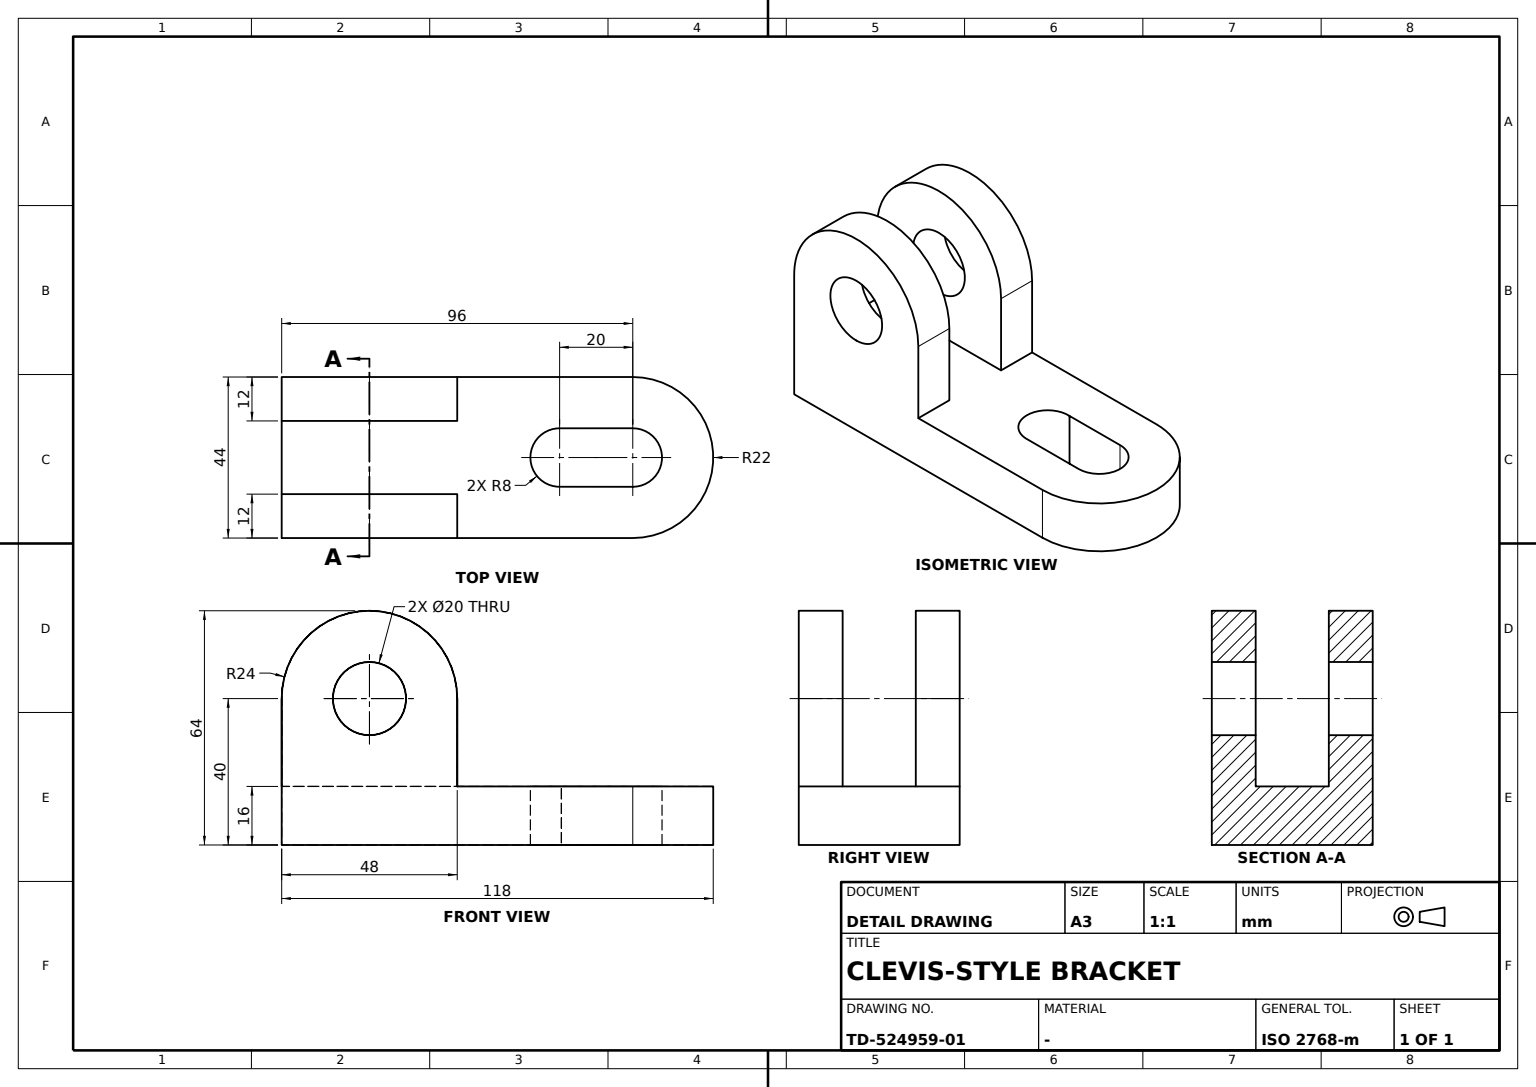
ISO-10303-21;
HEADER;
FILE_DESCRIPTION((''),'2;1');
FILE_NAME('','',(''),(''),'','','');
FILE_SCHEMA(('AUTOMOTIVE_DESIGN'));
ENDSEC;
DATA;
#1=APPLICATION_CONTEXT('');
#2=PRODUCT_CONTEXT('',#1,'mechanical');
#3=PRODUCT('','','',(#2));
#4=PRODUCT_DEFINITION_FORMATION('','',#3);
#5=PRODUCT_DEFINITION_CONTEXT('',#1,'design');
#6=PRODUCT_DEFINITION('','',#4,#5);
#7=PRODUCT_DEFINITION_SHAPE('','',#6);
#8=(LENGTH_UNIT()NAMED_UNIT(*)SI_UNIT(.MILLI.,.METRE.));
#9=(NAMED_UNIT(*)PLANE_ANGLE_UNIT()SI_UNIT($,.RADIAN.));
#10=(NAMED_UNIT(*)SI_UNIT($,.STERADIAN.)SOLID_ANGLE_UNIT());
#11=UNCERTAINTY_MEASURE_WITH_UNIT(LENGTH_MEASURE(0.005),#8,'distance_accuracy_value','');
#12=(GEOMETRIC_REPRESENTATION_CONTEXT(3)GLOBAL_UNCERTAINTY_ASSIGNED_CONTEXT((#11))GLOBAL_UNIT_ASSIGNED_CONTEXT((#8,#9,#10))REPRESENTATION_CONTEXT('',''));
#13=CARTESIAN_POINT('',(0.,-10.,40.));
#14=VERTEX_POINT('',#13);
#15=CARTESIAN_POINT('',(0.,-10.,16.));
#16=VERTEX_POINT('',#15);
#17=DIRECTION('',(0.,0.,-1.));
#18=VECTOR('',#17,1000.);
#19=LINE('',#13,#18);
#20=EDGE_CURVE('',#14,#16,#19,.T.);
#21=ORIENTED_EDGE('',*,*,#20,.F.);
#22=CARTESIAN_POINT('',(0.,-22.,40.));
#23=VERTEX_POINT('',#22);
#24=CARTESIAN_POINT('',(0.,16.,40.));
#25=DIRECTION('',(0.,1.,0.));
#26=VECTOR('',#25,1000.);
#27=LINE('',#24,#26);
#28=EDGE_CURVE('',#23,#14,#27,.T.);
#29=ORIENTED_EDGE('',*,*,#28,.F.);
#30=CARTESIAN_POINT('',(0.,-22.,16.));
#31=VERTEX_POINT('',#30);
#32=CARTESIAN_POINT('',(0.,-22.,0.));
#33=LINE('',#32,#18);
#34=EDGE_CURVE('',#23,#31,#33,.T.);
#35=ORIENTED_EDGE('',*,*,#34,.T.);
#36=CARTESIAN_POINT('',(0.,22.,16.));
#37=LINE('',#36,#26);
#38=EDGE_CURVE('',#31,#16,#37,.T.);
#39=ORIENTED_EDGE('',*,*,#38,.T.);
#40=EDGE_LOOP('',(#21,#29,#35,#39));
#41=FACE_BOUND('',#40,.T.);
#42=CARTESIAN_POINT('',(0.,22.,40.));
#43=DIRECTION('',(-1.,0.,0.));
#44=AXIS2_PLACEMENT_3D('',#42,#43,#17);
#45=PLANE('',#44);
#46=ADVANCED_FACE('',(#41),#45,.F.);
#47=CARTESIAN_POINT('',(-24.,10.,50.));
#48=VERTEX_POINT('',#47);
#49=CARTESIAN_POINT('',(-24.,10.,40.));
#50=DIRECTION('',(0.,0.,1.));
#51=AXIS2_PLACEMENT_3D('',#49,#25,#50);
#52=CIRCLE('',#51,10.);
#53=EDGE_CURVE('',#48,#48,#52,.T.);
#54=ORIENTED_EDGE('',*,*,#53,.T.);
#55=EDGE_LOOP('',(#54));
#56=FACE_BOUND('',#55,.T.);
#57=CARTESIAN_POINT('',(-48.,10.,16.));
#58=VERTEX_POINT('',#57);
#59=CARTESIAN_POINT('',(-48.,10.,40.));
#60=VERTEX_POINT('',#59);
#61=CARTESIAN_POINT('',(-48.,10.,0.));
#62=VECTOR('',#50,1000.);
#63=LINE('',#61,#62);
#64=EDGE_CURVE('',#58,#60,#63,.T.);
#65=ORIENTED_EDGE('',*,*,#64,.F.);
#66=CARTESIAN_POINT('',(0.,10.,16.));
#67=VERTEX_POINT('',#66);
#68=VECTOR('',#43,1000.);
#69=LINE('',#66,#68);
#70=EDGE_CURVE('',#67,#58,#69,.T.);
#71=ORIENTED_EDGE('',*,*,#70,.F.);
#72=CARTESIAN_POINT('',(0.,10.,40.));
#73=VERTEX_POINT('',#72);
#74=LINE('',#72,#18);
#75=EDGE_CURVE('',#73,#67,#74,.T.);
#76=ORIENTED_EDGE('',*,*,#75,.F.);
#77=CIRCLE('',#51,24.);
#78=EDGE_CURVE('',#60,#73,#77,.T.);
#79=ORIENTED_EDGE('',*,*,#78,.F.);
#80=EDGE_LOOP('',(#65,#71,#76,#79));
#81=FACE_BOUND('',#80,.T.);
#82=CARTESIAN_POINT('',(0.,10.,0.));
#83=AXIS2_PLACEMENT_3D('',#82,#25,#43);
#84=PLANE('',#83);
#85=ADVANCED_FACE('',(#56,#81),#84,.F.);
#86=CARTESIAN_POINT('',(48.,22.,0.));
#87=VERTEX_POINT('',#86);
#88=CARTESIAN_POINT('',(48.,22.,16.));
#89=VERTEX_POINT('',#88);
#90=CARTESIAN_POINT('',(48.,22.,8.));
#91=LINE('',#90,#62);
#92=EDGE_CURVE('',#87,#89,#91,.T.);
#93=ORIENTED_EDGE('',*,*,#92,.T.);
#94=CARTESIAN_POINT('',(48.,-22.,16.));
#95=VERTEX_POINT('',#94);
#96=CARTESIAN_POINT('',(48.,0.,16.));
#97=DIRECTION('',(1.,0.,0.));
#98=AXIS2_PLACEMENT_3D('',#96,#50,#97);
#99=CIRCLE('',#98,22.);
#100=EDGE_CURVE('',#95,#89,#99,.T.);
#101=ORIENTED_EDGE('',*,*,#100,.F.);
#102=CARTESIAN_POINT('',(48.,-22.,0.));
#103=VERTEX_POINT('',#102);
#104=CARTESIAN_POINT('',(48.,-22.,8.));
#105=LINE('',#104,#62);
#106=EDGE_CURVE('',#103,#95,#105,.T.);
#107=ORIENTED_EDGE('',*,*,#106,.F.);
#108=CARTESIAN_POINT('',(48.,0.,0.));
#109=AXIS2_PLACEMENT_3D('',#108,#50,#97);
#110=CIRCLE('',#109,22.);
#111=EDGE_CURVE('',#103,#87,#110,.T.);
#112=ORIENTED_EDGE('',*,*,#111,.T.);
#113=EDGE_LOOP('',(#93,#101,#107,#112));
#114=FACE_BOUND('',#113,.T.);
#115=CARTESIAN_POINT('',(48.,0.,8.));
#116=AXIS2_PLACEMENT_3D('',#115,#50,#97);
#117=CYLINDRICAL_SURFACE('',#116,22.);
#118=ADVANCED_FACE('',(#114),#117,.T.);
#119=ORIENTED_EDGE('',*,*,#92,.F.);
#120=CARTESIAN_POINT('',(-48.,22.,0.));
#121=VERTEX_POINT('',#120);
#122=CARTESIAN_POINT('',(0.,22.,0.));
#123=LINE('',#122,#68);
#124=EDGE_CURVE('',#87,#121,#123,.T.);
#125=ORIENTED_EDGE('',*,*,#124,.T.);
#126=CARTESIAN_POINT('',(-48.,22.,40.));
#127=VERTEX_POINT('',#126);
#128=LINE('',#120,#62);
#129=EDGE_CURVE('',#121,#127,#128,.T.);
#130=ORIENTED_EDGE('',*,*,#129,.T.);
#131=VERTEX_POINT('',#42);
#132=CARTESIAN_POINT('',(-24.,22.,40.));
#133=AXIS2_PLACEMENT_3D('',#132,#25,#50);
#134=CIRCLE('',#133,24.);
#135=EDGE_CURVE('',#127,#131,#134,.T.);
#136=ORIENTED_EDGE('',*,*,#135,.T.);
#137=VERTEX_POINT('',#36);
#138=LINE('',#42,#18);
#139=EDGE_CURVE('',#131,#137,#138,.T.);
#140=ORIENTED_EDGE('',*,*,#139,.T.);
#141=LINE('',#36,#68);
#142=EDGE_CURVE('',#89,#137,#141,.T.);
#143=ORIENTED_EDGE('',*,*,#142,.F.);
#144=EDGE_LOOP('',(#119,#125,#130,#136,#140,#143));
#145=FACE_BOUND('',#144,.T.);
#146=CARTESIAN_POINT('',(-24.,22.,50.));
#147=VERTEX_POINT('',#146);
#148=CIRCLE('',#133,10.);
#149=EDGE_CURVE('',#147,#147,#148,.T.);
#150=ORIENTED_EDGE('',*,*,#149,.F.);
#151=EDGE_LOOP('',(#150));
#152=FACE_BOUND('',#151,.T.);
#153=AXIS2_PLACEMENT_3D('',#86,#25,#43);
#154=PLANE('',#153);
#155=ADVANCED_FACE('',(#145,#152),#154,.T.);
#156=ORIENTED_EDGE('',*,*,#124,.F.);
#157=ORIENTED_EDGE('',*,*,#111,.F.);
#158=CARTESIAN_POINT('',(-48.,-22.,0.));
#159=VERTEX_POINT('',#158);
#160=VECTOR('',#97,1000.);
#161=LINE('',#32,#160);
#162=EDGE_CURVE('',#159,#103,#161,.T.);
#163=ORIENTED_EDGE('',*,*,#162,.F.);
#164=CARTESIAN_POINT('',(-48.,0.,0.));
#165=DIRECTION('',(0.,-1.,0.));
#166=VECTOR('',#165,1000.);
#167=LINE('',#164,#166);
#168=EDGE_CURVE('',#121,#159,#167,.T.);
#169=ORIENTED_EDGE('',*,*,#168,.F.);
#170=EDGE_LOOP('',(#156,#157,#163,#169));
#171=FACE_BOUND('',#170,.T.);
#172=CARTESIAN_POINT('',(28.487816,7.985113,0.));
#173=VERTEX_POINT('',#172);
#174=CARTESIAN_POINT('',(47.993896,7.999997,0.));
#175=VERTEX_POINT('',#174);
#176=CARTESIAN_POINT('',(-0.006076,7.963374,0.));
#177=DIRECTION('',(0.999999709,0.000762941,0.));
#178=VECTOR('',#177,1000.);
#179=LINE('',#176,#178);
#180=EDGE_CURVE('',#173,#175,#179,.T.);
#181=ORIENTED_EDGE('',*,*,#180,.F.);
#182=CARTESIAN_POINT('',(28.487816,-7.985113,0.));
#183=VERTEX_POINT('',#182);
#184=CARTESIAN_POINT('',(28.,0.,0.));
#185=AXIS2_PLACEMENT_3D('',#184,#50,#97);
#186=CIRCLE('',#185,8.);
#187=EDGE_CURVE('',#173,#183,#186,.T.);
#188=ORIENTED_EDGE('',*,*,#187,.T.);
#189=CARTESIAN_POINT('',(47.993896,-7.999997,0.));
#190=VERTEX_POINT('',#189);
#191=CARTESIAN_POINT('',(-0.006076,-7.963374,0.));
#192=DIRECTION('',(0.999999709,-0.000762941,0.));
#193=VECTOR('',#192,1000.);
#194=LINE('',#191,#193);
#195=EDGE_CURVE('',#183,#190,#194,.T.);
#196=ORIENTED_EDGE('',*,*,#195,.T.);
#197=CIRCLE('',#109,8.);
#198=EDGE_CURVE('',#190,#175,#197,.T.);
#199=ORIENTED_EDGE('',*,*,#198,.T.);
#200=EDGE_LOOP('',(#181,#188,#196,#199));
#201=FACE_BOUND('',#200,.T.);
#202=CARTESIAN_POINT('',(0.,0.,0.));
#203=AXIS2_PLACEMENT_3D('',#202,#50,#97);
#204=PLANE('',#203);
#205=ADVANCED_FACE('',(#171,#201),#204,.F.);
#206=CARTESIAN_POINT('',(-24.,-10.,50.));
#207=VERTEX_POINT('',#206);
#208=CARTESIAN_POINT('',(-24.,-10.,40.));
#209=AXIS2_PLACEMENT_3D('',#208,#25,#50);
#210=CIRCLE('',#209,10.);
#211=EDGE_CURVE('',#207,#207,#210,.T.);
#212=ORIENTED_EDGE('',*,*,#211,.F.);
#213=EDGE_LOOP('',(#212));
#214=FACE_BOUND('',#213,.T.);
#215=CARTESIAN_POINT('',(-48.,-10.,40.));
#216=VERTEX_POINT('',#215);
#217=CIRCLE('',#209,24.);
#218=EDGE_CURVE('',#216,#14,#217,.T.);
#219=ORIENTED_EDGE('',*,*,#218,.T.);
#220=ORIENTED_EDGE('',*,*,#20,.T.);
#221=CARTESIAN_POINT('',(-48.,-10.,16.));
#222=VERTEX_POINT('',#221);
#223=LINE('',#15,#68);
#224=EDGE_CURVE('',#16,#222,#223,.T.);
#225=ORIENTED_EDGE('',*,*,#224,.T.);
#226=CARTESIAN_POINT('',(-48.,-10.,0.));
#227=LINE('',#226,#62);
#228=EDGE_CURVE('',#222,#216,#227,.T.);
#229=ORIENTED_EDGE('',*,*,#228,.T.);
#230=EDGE_LOOP('',(#219,#220,#225,#229));
#231=FACE_BOUND('',#230,.T.);
#232=CARTESIAN_POINT('',(0.,-10.,0.));
#233=AXIS2_PLACEMENT_3D('',#232,#25,#43);
#234=PLANE('',#233);
#235=ADVANCED_FACE('',(#214,#231),#234,.T.);
#236=ORIENTED_EDGE('',*,*,#149,.T.);
#237=EDGE_LOOP('',(#236));
#238=FACE_BOUND('',#237,.T.);
#239=ORIENTED_EDGE('',*,*,#53,.F.);
#240=EDGE_LOOP('',(#239));
#241=FACE_BOUND('',#240,.T.);
#242=CARTESIAN_POINT('',(-24.,16.,40.));
#243=AXIS2_PLACEMENT_3D('',#242,#25,#43);
#244=CYLINDRICAL_SURFACE('',#243,10.);
#245=ADVANCED_FACE('',(#238,#241),#244,.F.);
#246=CARTESIAN_POINT('',(47.993896,-7.999997,16.));
#247=VERTEX_POINT('',#246);
#248=CARTESIAN_POINT('',(47.993896,-7.999997,8.));
#249=LINE('',#248,#62);
#250=EDGE_CURVE('',#190,#247,#249,.T.);
#251=ORIENTED_EDGE('',*,*,#250,.T.);
#252=CARTESIAN_POINT('',(47.993896,7.999997,16.));
#253=VERTEX_POINT('',#252);
#254=CIRCLE('',#98,8.);
#255=EDGE_CURVE('',#247,#253,#254,.T.);
#256=ORIENTED_EDGE('',*,*,#255,.T.);
#257=CARTESIAN_POINT('',(47.993896,7.999997,8.));
#258=LINE('',#257,#62);
#259=EDGE_CURVE('',#175,#253,#258,.T.);
#260=ORIENTED_EDGE('',*,*,#259,.F.);
#261=ORIENTED_EDGE('',*,*,#198,.F.);
#262=EDGE_LOOP('',(#251,#256,#260,#261));
#263=FACE_BOUND('',#262,.T.);
#264=CYLINDRICAL_SURFACE('',#116,8.);
#265=ADVANCED_FACE('',(#263),#264,.F.);
#266=CARTESIAN_POINT('',(28.487816,7.985113,16.));
#267=VERTEX_POINT('',#266);
#268=CARTESIAN_POINT('',(-0.006076,7.963374,16.));
#269=LINE('',#268,#178);
#270=EDGE_CURVE('',#267,#253,#269,.T.);
#271=ORIENTED_EDGE('',*,*,#270,.T.);
#272=ORIENTED_EDGE('',*,*,#255,.F.);
#273=CARTESIAN_POINT('',(28.487816,-7.985113,16.));
#274=VERTEX_POINT('',#273);
#275=CARTESIAN_POINT('',(-0.006076,-7.963374,16.));
#276=LINE('',#275,#193);
#277=EDGE_CURVE('',#274,#247,#276,.T.);
#278=ORIENTED_EDGE('',*,*,#277,.F.);
#279=CARTESIAN_POINT('',(28.,0.,16.));
#280=AXIS2_PLACEMENT_3D('',#279,#50,#97);
#281=CIRCLE('',#280,8.);
#282=EDGE_CURVE('',#267,#274,#281,.T.);
#283=ORIENTED_EDGE('',*,*,#282,.F.);
#284=EDGE_LOOP('',(#271,#272,#278,#283));
#285=FACE_BOUND('',#284,.T.);
#286=ORIENTED_EDGE('',*,*,#70,.T.);
#287=CARTESIAN_POINT('',(-48.,0.,16.));
#288=LINE('',#287,#166);
#289=EDGE_CURVE('',#58,#222,#288,.T.);
#290=ORIENTED_EDGE('',*,*,#289,.T.);
#291=ORIENTED_EDGE('',*,*,#224,.F.);
#292=ORIENTED_EDGE('',*,*,#38,.F.);
#293=LINE('',#30,#160);
#294=EDGE_CURVE('',#31,#95,#293,.T.);
#295=ORIENTED_EDGE('',*,*,#294,.T.);
#296=ORIENTED_EDGE('',*,*,#100,.T.);
#297=ORIENTED_EDGE('',*,*,#142,.T.);
#298=CARTESIAN_POINT('',(0.,0.,16.));
#299=LINE('',#298,#166);
#300=EDGE_CURVE('',#137,#67,#299,.T.);
#301=ORIENTED_EDGE('',*,*,#300,.T.);
#302=EDGE_LOOP('',(#286,#290,#291,#292,#295,#296,#297,#301));
#303=FACE_BOUND('',#302,.T.);
#304=AXIS2_PLACEMENT_3D('',#298,#50,#97);
#305=PLANE('',#304);
#306=ADVANCED_FACE('',(#285,#303),#305,.T.);
#307=CARTESIAN_POINT('',(-24.,-22.,30.));
#308=VERTEX_POINT('',#307);
#309=CARTESIAN_POINT('',(-24.,-22.,40.));
#310=AXIS2_PLACEMENT_3D('',#309,#165,#17);
#311=CIRCLE('',#310,10.);
#312=EDGE_CURVE('',#308,#308,#311,.F.);
#313=ORIENTED_EDGE('',*,*,#312,.F.);
#314=EDGE_LOOP('',(#313));
#315=FACE_BOUND('',#314,.T.);
#316=ORIENTED_EDGE('',*,*,#211,.T.);
#317=EDGE_LOOP('',(#316));
#318=FACE_BOUND('',#317,.T.);
#319=ADVANCED_FACE('',(#315,#318),#244,.F.);
#320=ORIENTED_EDGE('',*,*,#75,.T.);
#321=ORIENTED_EDGE('',*,*,#300,.F.);
#322=ORIENTED_EDGE('',*,*,#139,.F.);
#323=EDGE_CURVE('',#131,#73,#27,.F.);
#324=ORIENTED_EDGE('',*,*,#323,.T.);
#325=EDGE_LOOP('',(#320,#321,#322,#324));
#326=FACE_BOUND('',#325,.T.);
#327=ADVANCED_FACE('',(#326),#45,.F.);
#328=CARTESIAN_POINT('',(-48.,16.,40.));
#329=LINE('',#328,#26);
#330=EDGE_CURVE('',#127,#60,#329,.F.);
#331=ORIENTED_EDGE('',*,*,#330,.T.);
#332=ORIENTED_EDGE('',*,*,#78,.T.);
#333=ORIENTED_EDGE('',*,*,#323,.F.);
#334=ORIENTED_EDGE('',*,*,#135,.F.);
#335=EDGE_LOOP('',(#331,#332,#333,#334));
#336=FACE_BOUND('',#335,.T.);
#337=CYLINDRICAL_SURFACE('',#243,24.);
#338=ADVANCED_FACE('',(#336),#337,.T.);
#339=ORIENTED_EDGE('',*,*,#129,.F.);
#340=ORIENTED_EDGE('',*,*,#168,.T.);
#341=CARTESIAN_POINT('',(-48.,-22.,40.));
#342=VERTEX_POINT('',#341);
#343=LINE('',#158,#62);
#344=EDGE_CURVE('',#159,#342,#343,.T.);
#345=ORIENTED_EDGE('',*,*,#344,.T.);
#346=EDGE_CURVE('',#342,#216,#329,.T.);
#347=ORIENTED_EDGE('',*,*,#346,.T.);
#348=ORIENTED_EDGE('',*,*,#228,.F.);
#349=ORIENTED_EDGE('',*,*,#289,.F.);
#350=ORIENTED_EDGE('',*,*,#64,.T.);
#351=ORIENTED_EDGE('',*,*,#330,.F.);
#352=EDGE_LOOP('',(#339,#340,#345,#347,#348,#349,#350,#351));
#353=FACE_BOUND('',#352,.T.);
#354=AXIS2_PLACEMENT_3D('',#120,#43,#165);
#355=PLANE('',#354);
#356=ADVANCED_FACE('',(#353),#355,.T.);
#357=CIRCLE('',#310,24.);
#358=EDGE_CURVE('',#342,#23,#357,.F.);
#359=ORIENTED_EDGE('',*,*,#358,.F.);
#360=ORIENTED_EDGE('',*,*,#344,.F.);
#361=ORIENTED_EDGE('',*,*,#162,.T.);
#362=ORIENTED_EDGE('',*,*,#106,.T.);
#363=ORIENTED_EDGE('',*,*,#294,.F.);
#364=ORIENTED_EDGE('',*,*,#34,.F.);
#365=EDGE_LOOP('',(#359,#360,#361,#362,#363,#364));
#366=FACE_BOUND('',#365,.T.);
#367=ORIENTED_EDGE('',*,*,#312,.T.);
#368=EDGE_LOOP('',(#367));
#369=FACE_BOUND('',#368,.T.);
#370=AXIS2_PLACEMENT_3D('',#158,#165,#97);
#371=PLANE('',#370);
#372=ADVANCED_FACE('',(#366,#369),#371,.T.);
#373=ORIENTED_EDGE('',*,*,#277,.T.);
#374=ORIENTED_EDGE('',*,*,#250,.F.);
#375=ORIENTED_EDGE('',*,*,#195,.F.);
#376=LINE('',#182,#62);
#377=EDGE_CURVE('',#183,#274,#376,.T.);
#378=ORIENTED_EDGE('',*,*,#377,.T.);
#379=EDGE_LOOP('',(#373,#374,#375,#378));
#380=FACE_BOUND('',#379,.T.);
#381=DIRECTION('',(-0.000762941,-0.999999709,0.));
#382=AXIS2_PLACEMENT_3D('',#182,#381,#192);
#383=PLANE('',#382);
#384=ADVANCED_FACE('',(#380),#383,.F.);
#385=ORIENTED_EDGE('',*,*,#259,.T.);
#386=ORIENTED_EDGE('',*,*,#270,.F.);
#387=LINE('',#172,#62);
#388=EDGE_CURVE('',#173,#267,#387,.T.);
#389=ORIENTED_EDGE('',*,*,#388,.F.);
#390=ORIENTED_EDGE('',*,*,#180,.T.);
#391=EDGE_LOOP('',(#385,#386,#389,#390));
#392=FACE_BOUND('',#391,.T.);
#393=DIRECTION('',(0.000762941,-0.999999709,0.));
#394=AXIS2_PLACEMENT_3D('',#172,#393,#177);
#395=PLANE('',#394);
#396=ADVANCED_FACE('',(#392),#395,.T.);
#397=ORIENTED_EDGE('',*,*,#346,.F.);
#398=ORIENTED_EDGE('',*,*,#358,.T.);
#399=ORIENTED_EDGE('',*,*,#28,.T.);
#400=ORIENTED_EDGE('',*,*,#218,.F.);
#401=EDGE_LOOP('',(#397,#398,#399,#400));
#402=FACE_BOUND('',#401,.T.);
#403=ADVANCED_FACE('',(#402),#337,.T.);
#404=ORIENTED_EDGE('',*,*,#377,.F.);
#405=ORIENTED_EDGE('',*,*,#187,.F.);
#406=ORIENTED_EDGE('',*,*,#388,.T.);
#407=ORIENTED_EDGE('',*,*,#282,.T.);
#408=EDGE_LOOP('',(#404,#405,#406,#407));
#409=FACE_BOUND('',#408,.T.);
#410=CARTESIAN_POINT('',(28.,0.,8.));
#411=AXIS2_PLACEMENT_3D('',#410,#50,#97);
#412=CYLINDRICAL_SURFACE('',#411,8.);
#413=ADVANCED_FACE('',(#409),#412,.F.);
#414=CLOSED_SHELL('',(#46,#85,#118,#155,#205,#235,#245,#265,#306,#319,#327,#338,#356,#372,#384,#396,#403,#413));
#415=MANIFOLD_SOLID_BREP('',#414);
#416=ADVANCED_BREP_SHAPE_REPRESENTATION('',(#415),#12);
#417=SHAPE_DEFINITION_REPRESENTATION(#7,#416);
ENDSEC;
END-ISO-10303-21;
